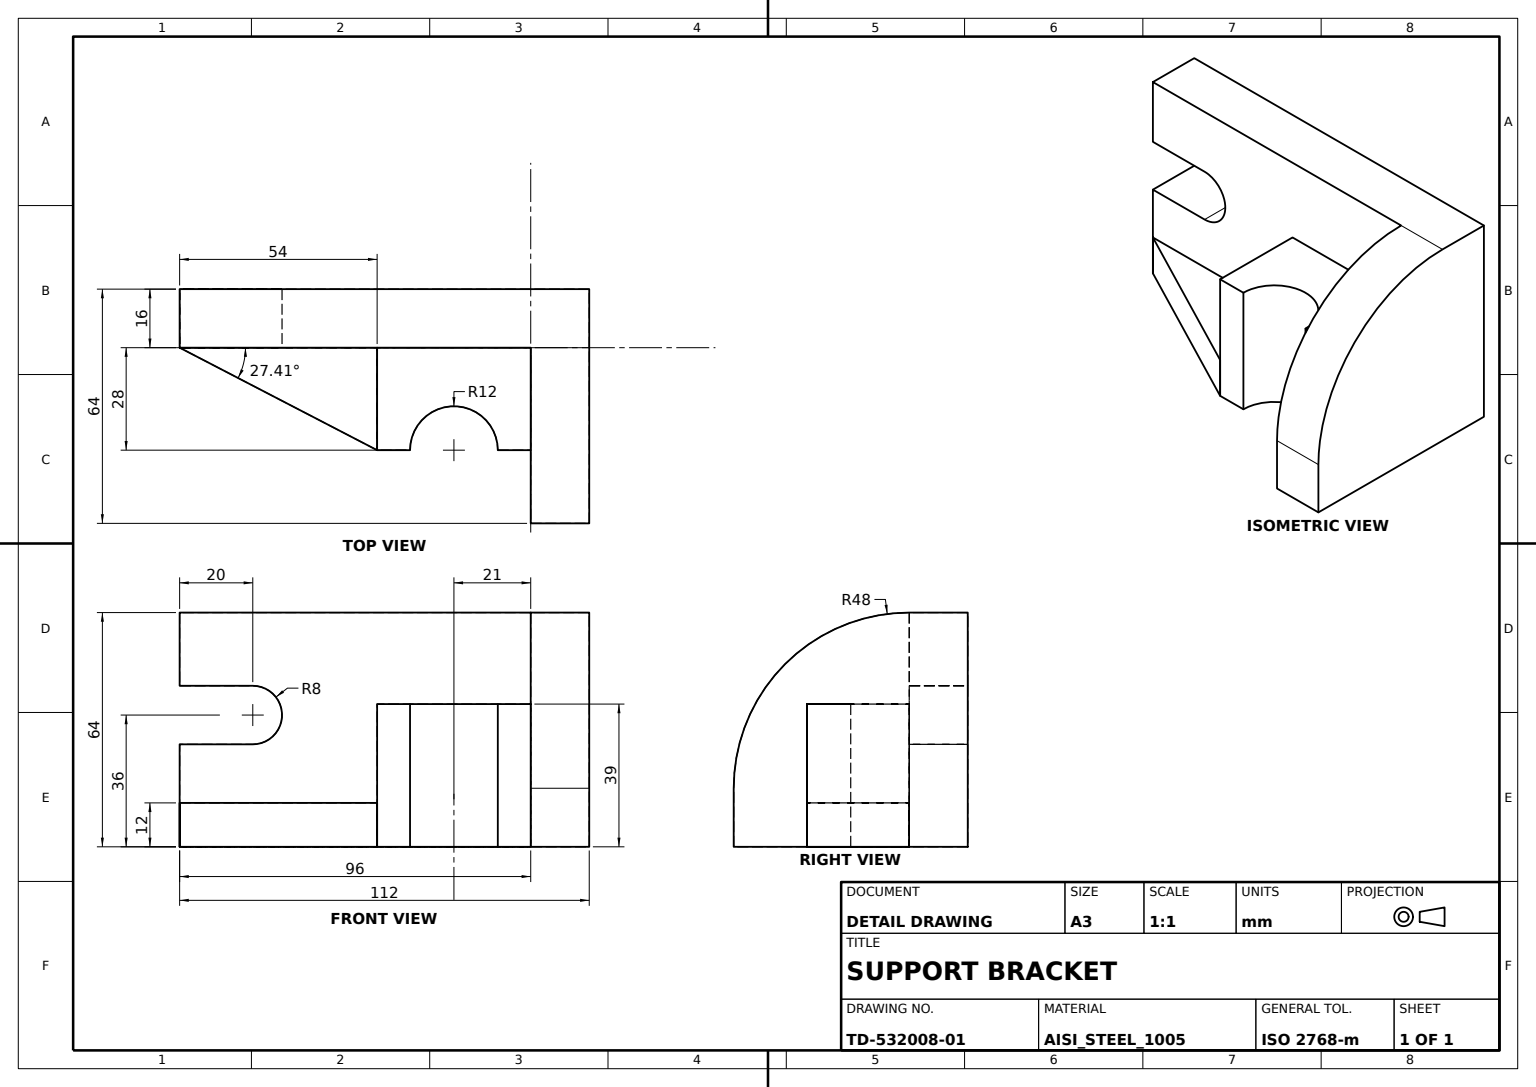
ISO-10303-21;
HEADER;
FILE_DESCRIPTION((''),'2;1');
FILE_NAME('','',(''),(''),'','','');
FILE_SCHEMA(('AUTOMOTIVE_DESIGN'));
ENDSEC;
DATA;
#1=APPLICATION_CONTEXT('');
#2=PRODUCT_CONTEXT('',#1,'mechanical');
#3=PRODUCT('','','',(#2));
#4=PRODUCT_DEFINITION_FORMATION('','',#3);
#5=PRODUCT_DEFINITION_CONTEXT('',#1,'design');
#6=PRODUCT_DEFINITION('','',#4,#5);
#7=PRODUCT_DEFINITION_SHAPE('','',#6);
#8=(LENGTH_UNIT()NAMED_UNIT(*)SI_UNIT(.MILLI.,.METRE.));
#9=(NAMED_UNIT(*)PLANE_ANGLE_UNIT()SI_UNIT($,.RADIAN.));
#10=(NAMED_UNIT(*)SI_UNIT($,.STERADIAN.)SOLID_ANGLE_UNIT());
#11=UNCERTAINTY_MEASURE_WITH_UNIT(LENGTH_MEASURE(0.005),#8,'distance_accuracy_value','');
#12=(GEOMETRIC_REPRESENTATION_CONTEXT(3)GLOBAL_UNCERTAINTY_ASSIGNED_CONTEXT((#11))GLOBAL_UNIT_ASSIGNED_CONTEXT((#8,#9,#10))REPRESENTATION_CONTEXT('',''));
#13=CARTESIAN_POINT('',(16.,0.,64.));
#14=VERTEX_POINT('',#13);
#15=CARTESIAN_POINT('',(0.,0.,64.));
#16=VERTEX_POINT('',#15);
#17=DIRECTION('',(-1.,0.,0.));
#18=VECTOR('',#17,1000.);
#19=LINE('',#13,#18);
#20=EDGE_CURVE('',#14,#16,#19,.T.);
#21=ORIENTED_EDGE('',*,*,#20,.T.);
#22=CARTESIAN_POINT('',(0.,0.,44.));
#23=VERTEX_POINT('',#22);
#24=CARTESIAN_POINT('',(0.,0.,0.));
#25=DIRECTION('',(0.,0.,1.));
#26=VECTOR('',#25,1000.);
#27=LINE('',#24,#26);
#28=EDGE_CURVE('',#23,#16,#27,.T.);
#29=ORIENTED_EDGE('',*,*,#28,.F.);
#30=CARTESIAN_POINT('',(16.,0.,44.));
#31=VERTEX_POINT('',#30);
#32=DIRECTION('',(1.,0.,0.));
#33=VECTOR('',#32,1000.);
#34=LINE('',#22,#33);
#35=EDGE_CURVE('',#23,#31,#34,.T.);
#36=ORIENTED_EDGE('',*,*,#35,.T.);
#37=CARTESIAN_POINT('',(16.,0.,0.));
#38=LINE('',#37,#26);
#39=EDGE_CURVE('',#31,#14,#38,.T.);
#40=ORIENTED_EDGE('',*,*,#39,.T.);
#41=EDGE_LOOP('',(#21,#29,#36,#40));
#42=FACE_BOUND('',#41,.T.);
#43=DIRECTION('',(0.,-1.,0.));
#44=DIRECTION('',(0.,0.,-1.));
#45=AXIS2_PLACEMENT_3D('',#37,#43,#44);
#46=PLANE('',#45);
#47=ADVANCED_FACE('',(#42),#46,.T.);
#48=CARTESIAN_POINT('',(64.,112.,0.));
#49=VERTEX_POINT('',#48);
#50=CARTESIAN_POINT('',(0.,112.,0.));
#51=VERTEX_POINT('',#50);
#52=LINE('',#48,#18);
#53=EDGE_CURVE('',#49,#51,#52,.T.);
#54=ORIENTED_EDGE('',*,*,#53,.F.);
#55=CARTESIAN_POINT('',(64.,96.,0.));
#56=VERTEX_POINT('',#55);
#57=VECTOR('',#43,1000.);
#58=LINE('',#48,#57);
#59=EDGE_CURVE('',#49,#56,#58,.T.);
#60=ORIENTED_EDGE('',*,*,#59,.T.);
#61=CARTESIAN_POINT('',(16.,96.,0.));
#62=VERTEX_POINT('',#61);
#63=LINE('',#55,#18);
#64=EDGE_CURVE('',#56,#62,#63,.T.);
#65=ORIENTED_EDGE('',*,*,#64,.T.);
#66=VERTEX_POINT('',#37);
#67=LINE('',#61,#57);
#68=EDGE_CURVE('',#62,#66,#67,.T.);
#69=ORIENTED_EDGE('',*,*,#68,.T.);
#70=VERTEX_POINT('',#24);
#71=LINE('',#37,#18);
#72=EDGE_CURVE('',#66,#70,#71,.T.);
#73=ORIENTED_EDGE('',*,*,#72,.T.);
#74=CARTESIAN_POINT('',(0.,96.,0.));
#75=LINE('',#74,#57);
#76=EDGE_CURVE('',#51,#70,#75,.T.);
#77=ORIENTED_EDGE('',*,*,#76,.F.);
#78=EDGE_LOOP('',(#54,#60,#65,#69,#73,#77));
#79=FACE_BOUND('',#78,.T.);
#80=AXIS2_PLACEMENT_3D('',#61,#44,#17);
#81=PLANE('',#80);
#82=ADVANCED_FACE('',(#79),#81,.T.);
#83=CARTESIAN_POINT('',(16.,20.,44.));
#84=VERTEX_POINT('',#83);
#85=LINE('',#83,#57);
#86=EDGE_CURVE('',#84,#31,#85,.T.);
#87=ORIENTED_EDGE('',*,*,#86,.T.);
#88=ORIENTED_EDGE('',*,*,#35,.F.);
#89=CARTESIAN_POINT('',(0.,20.,44.));
#90=VERTEX_POINT('',#89);
#91=LINE('',#89,#57);
#92=EDGE_CURVE('',#90,#23,#91,.T.);
#93=ORIENTED_EDGE('',*,*,#92,.F.);
#94=LINE('',#89,#33);
#95=EDGE_CURVE('',#84,#90,#94,.F.);
#96=ORIENTED_EDGE('',*,*,#95,.F.);
#97=EDGE_LOOP('',(#87,#88,#93,#96));
#98=FACE_BOUND('',#97,.T.);
#99=AXIS2_PLACEMENT_3D('',#89,#25,#32);
#100=PLANE('',#99);
#101=ADVANCED_FACE('',(#98),#100,.F.);
#102=CARTESIAN_POINT('',(16.,20.,28.));
#103=VERTEX_POINT('',#102);
#104=CARTESIAN_POINT('',(16.,20.,36.));
#105=AXIS2_PLACEMENT_3D('',#104,#32,#43);
#106=CIRCLE('',#105,8.);
#107=EDGE_CURVE('',#103,#84,#106,.T.);
#108=ORIENTED_EDGE('',*,*,#107,.F.);
#109=CARTESIAN_POINT('',(16.,0.,28.));
#110=VERTEX_POINT('',#109);
#111=DIRECTION('',(0.,1.,0.));
#112=VECTOR('',#111,1000.);
#113=LINE('',#109,#112);
#114=EDGE_CURVE('',#110,#103,#113,.T.);
#115=ORIENTED_EDGE('',*,*,#114,.F.);
#116=EDGE_CURVE('',#66,#110,#38,.T.);
#117=ORIENTED_EDGE('',*,*,#116,.F.);
#118=ORIENTED_EDGE('',*,*,#68,.F.);
#119=CARTESIAN_POINT('',(16.,96.,64.));
#120=VERTEX_POINT('',#119);
#121=VECTOR('',#44,1000.);
#122=LINE('',#119,#121);
#123=EDGE_CURVE('',#120,#62,#122,.T.);
#124=ORIENTED_EDGE('',*,*,#123,.F.);
#125=LINE('',#13,#112);
#126=EDGE_CURVE('',#14,#120,#125,.T.);
#127=ORIENTED_EDGE('',*,*,#126,.F.);
#128=ORIENTED_EDGE('',*,*,#39,.F.);
#129=ORIENTED_EDGE('',*,*,#86,.F.);
#130=EDGE_LOOP('',(#108,#115,#117,#118,#124,#127,#128,#129));
#131=FACE_BOUND('',#130,.T.);
#132=AXIS2_PLACEMENT_3D('',#37,#17,#25);
#133=PLANE('',#132);
#134=ADVANCED_FACE('',(#131),#133,.F.);
#135=CARTESIAN_POINT('',(0.,0.,28.));
#136=VERTEX_POINT('',#135);
#137=EDGE_CURVE('',#70,#136,#27,.T.);
#138=ORIENTED_EDGE('',*,*,#137,.F.);
#139=ORIENTED_EDGE('',*,*,#72,.F.);
#140=ORIENTED_EDGE('',*,*,#116,.T.);
#141=LINE('',#135,#33);
#142=EDGE_CURVE('',#136,#110,#141,.T.);
#143=ORIENTED_EDGE('',*,*,#142,.F.);
#144=EDGE_LOOP('',(#138,#139,#140,#143));
#145=FACE_BOUND('',#144,.T.);
#146=ADVANCED_FACE('',(#145),#46,.T.);
#147=ORIENTED_EDGE('',*,*,#123,.T.);
#148=ORIENTED_EDGE('',*,*,#64,.F.);
#149=CARTESIAN_POINT('',(64.,96.,16.));
#150=VERTEX_POINT('',#149);
#151=CARTESIAN_POINT('',(64.,96.,64.));
#152=LINE('',#151,#121);
#153=EDGE_CURVE('',#150,#56,#152,.T.);
#154=ORIENTED_EDGE('',*,*,#153,.F.);
#155=CARTESIAN_POINT('',(16.,96.,16.));
#156=AXIS2_PLACEMENT_3D('',#155,#111,#25);
#157=CIRCLE('',#156,48.);
#158=EDGE_CURVE('',#150,#120,#157,.F.);
#159=ORIENTED_EDGE('',*,*,#158,.T.);
#160=EDGE_LOOP('',(#147,#148,#154,#159));
#161=FACE_BOUND('',#160,.T.);
#162=AXIS2_PLACEMENT_3D('',#74,#111,#25);
#163=PLANE('',#162);
#164=ADVANCED_FACE('',(#161),#163,.F.);
#165=ORIENTED_EDGE('',*,*,#59,.F.);
#166=CARTESIAN_POINT('',(64.,112.,16.));
#167=VERTEX_POINT('',#166);
#168=CARTESIAN_POINT('',(64.,112.,64.));
#169=LINE('',#168,#121);
#170=EDGE_CURVE('',#167,#49,#169,.T.);
#171=ORIENTED_EDGE('',*,*,#170,.F.);
#172=LINE('',#149,#57);
#173=EDGE_CURVE('',#167,#150,#172,.T.);
#174=ORIENTED_EDGE('',*,*,#173,.T.);
#175=ORIENTED_EDGE('',*,*,#153,.T.);
#176=EDGE_LOOP('',(#165,#171,#174,#175));
#177=FACE_BOUND('',#176,.T.);
#178=AXIS2_PLACEMENT_3D('',#168,#17,#25);
#179=PLANE('',#178);
#180=ADVANCED_FACE('',(#177),#179,.F.);
#181=ORIENTED_EDGE('',*,*,#142,.T.);
#182=ORIENTED_EDGE('',*,*,#114,.T.);
#183=CARTESIAN_POINT('',(0.,20.,28.));
#184=VERTEX_POINT('',#183);
#185=LINE('',#183,#33);
#186=EDGE_CURVE('',#103,#184,#185,.F.);
#187=ORIENTED_EDGE('',*,*,#186,.T.);
#188=LINE('',#135,#112);
#189=EDGE_CURVE('',#136,#184,#188,.T.);
#190=ORIENTED_EDGE('',*,*,#189,.F.);
#191=EDGE_LOOP('',(#181,#182,#187,#190));
#192=FACE_BOUND('',#191,.T.);
#193=AXIS2_PLACEMENT_3D('',#135,#44,#111);
#194=PLANE('',#193);
#195=ADVANCED_FACE('',(#192),#194,.F.);
#196=CARTESIAN_POINT('',(16.,112.,64.));
#197=VERTEX_POINT('',#196);
#198=LINE('',#196,#57);
#199=EDGE_CURVE('',#120,#197,#198,.F.);
#200=ORIENTED_EDGE('',*,*,#199,.F.);
#201=ORIENTED_EDGE('',*,*,#158,.F.);
#202=ORIENTED_EDGE('',*,*,#173,.F.);
#203=CARTESIAN_POINT('',(16.,112.,16.));
#204=AXIS2_PLACEMENT_3D('',#203,#111,#25);
#205=CIRCLE('',#204,48.);
#206=EDGE_CURVE('',#197,#167,#205,.T.);
#207=ORIENTED_EDGE('',*,*,#206,.F.);
#208=EDGE_LOOP('',(#200,#201,#202,#207));
#209=FACE_BOUND('',#208,.T.);
#210=CYLINDRICAL_SURFACE('',#204,48.);
#211=ADVANCED_FACE('',(#209),#210,.T.);
#212=ORIENTED_EDGE('',*,*,#170,.T.);
#213=ORIENTED_EDGE('',*,*,#53,.T.);
#214=CARTESIAN_POINT('',(0.,112.,64.));
#215=VERTEX_POINT('',#214);
#216=LINE('',#50,#26);
#217=EDGE_CURVE('',#51,#215,#216,.T.);
#218=ORIENTED_EDGE('',*,*,#217,.T.);
#219=LINE('',#214,#33);
#220=EDGE_CURVE('',#215,#197,#219,.T.);
#221=ORIENTED_EDGE('',*,*,#220,.T.);
#222=ORIENTED_EDGE('',*,*,#206,.T.);
#223=EDGE_LOOP('',(#212,#213,#218,#221,#222));
#224=FACE_BOUND('',#223,.T.);
#225=AXIS2_PLACEMENT_3D('',#50,#111,#25);
#226=PLANE('',#225);
#227=ADVANCED_FACE('',(#224),#226,.T.);
#228=ORIENTED_EDGE('',*,*,#220,.F.);
#229=LINE('',#15,#112);
#230=EDGE_CURVE('',#16,#215,#229,.T.);
#231=ORIENTED_EDGE('',*,*,#230,.F.);
#232=ORIENTED_EDGE('',*,*,#20,.F.);
#233=ORIENTED_EDGE('',*,*,#126,.T.);
#234=ORIENTED_EDGE('',*,*,#199,.T.);
#235=EDGE_LOOP('',(#228,#231,#232,#233,#234));
#236=FACE_BOUND('',#235,.T.);
#237=AXIS2_PLACEMENT_3D('',#13,#25,#43);
#238=PLANE('',#237);
#239=ADVANCED_FACE('',(#236),#238,.T.);
#240=ORIENTED_EDGE('',*,*,#230,.T.);
#241=ORIENTED_EDGE('',*,*,#217,.F.);
#242=ORIENTED_EDGE('',*,*,#76,.T.);
#243=ORIENTED_EDGE('',*,*,#137,.T.);
#244=ORIENTED_EDGE('',*,*,#189,.T.);
#245=CARTESIAN_POINT('',(0.,20.,36.));
#246=AXIS2_PLACEMENT_3D('',#245,#32,#43);
#247=CIRCLE('',#246,8.);
#248=EDGE_CURVE('',#184,#90,#247,.T.);
#249=ORIENTED_EDGE('',*,*,#248,.T.);
#250=ORIENTED_EDGE('',*,*,#92,.T.);
#251=ORIENTED_EDGE('',*,*,#28,.T.);
#252=EDGE_LOOP('',(#240,#241,#242,#243,#244,#249,#250,#251));
#253=FACE_BOUND('',#252,.T.);
#254=AXIS2_PLACEMENT_3D('',#24,#17,#25);
#255=PLANE('',#254);
#256=ADVANCED_FACE('',(#253),#255,.T.);
#257=ORIENTED_EDGE('',*,*,#186,.F.);
#258=ORIENTED_EDGE('',*,*,#107,.T.);
#259=ORIENTED_EDGE('',*,*,#95,.T.);
#260=ORIENTED_EDGE('',*,*,#248,.F.);
#261=EDGE_LOOP('',(#257,#258,#259,#260));
#262=FACE_BOUND('',#261,.T.);
#263=AXIS2_PLACEMENT_3D('',#245,#32,#44);
#264=CYLINDRICAL_SURFACE('',#263,8.);
#265=ADVANCED_FACE('',(#262),#264,.F.);
#266=CLOSED_SHELL('',(#47,#82,#101,#134,#146,#164,#180,#195,#211,#227,#239,#256,#265));
#267=MANIFOLD_SOLID_BREP('',#266);
#268=CARTESIAN_POINT('',(16.,54.,0.));
#269=VERTEX_POINT('',#268);
#270=VERTEX_POINT('',#61);
#271=LINE('',#268,#112);
#272=EDGE_CURVE('',#269,#270,#271,.T.);
#273=ORIENTED_EDGE('',*,*,#272,.T.);
#274=CARTESIAN_POINT('',(44.,96.,0.));
#275=VERTEX_POINT('',#274);
#276=LINE('',#274,#18);
#277=EDGE_CURVE('',#275,#270,#276,.T.);
#278=ORIENTED_EDGE('',*,*,#277,.F.);
#279=CARTESIAN_POINT('',(44.,87.,0.));
#280=VERTEX_POINT('',#279);
#281=CARTESIAN_POINT('',(44.,54.,0.));
#282=LINE('',#281,#112);
#283=EDGE_CURVE('',#280,#275,#282,.T.);
#284=ORIENTED_EDGE('',*,*,#283,.F.);
#285=CARTESIAN_POINT('',(44.,63.,0.));
#286=VERTEX_POINT('',#285);
#287=CARTESIAN_POINT('',(44.,75.,0.));
#288=AXIS2_PLACEMENT_3D('',#287,#25,#32);
#289=CIRCLE('',#288,12.);
#290=EDGE_CURVE('',#286,#280,#289,.F.);
#291=ORIENTED_EDGE('',*,*,#290,.F.);
#292=VERTEX_POINT('',#281);
#293=EDGE_CURVE('',#292,#286,#282,.T.);
#294=ORIENTED_EDGE('',*,*,#293,.F.);
#295=LINE('',#281,#18);
#296=EDGE_CURVE('',#292,#269,#295,.T.);
#297=ORIENTED_EDGE('',*,*,#296,.T.);
#298=EDGE_LOOP('',(#273,#278,#284,#291,#294,#297));
#299=FACE_BOUND('',#298,.T.);
#300=AXIS2_PLACEMENT_3D('',#281,#25,#32);
#301=PLANE('',#300);
#302=ADVANCED_FACE('',(#299),#301,.F.);
#303=CARTESIAN_POINT('',(44.,63.,39.));
#304=VERTEX_POINT('',#303);
#305=CARTESIAN_POINT('',(44.,54.,39.));
#306=VERTEX_POINT('',#305);
#307=CARTESIAN_POINT('',(44.,96.,39.));
#308=LINE('',#307,#57);
#309=EDGE_CURVE('',#304,#306,#308,.T.);
#310=ORIENTED_EDGE('',*,*,#309,.T.);
#311=LINE('',#305,#121);
#312=EDGE_CURVE('',#306,#292,#311,.T.);
#313=ORIENTED_EDGE('',*,*,#312,.T.);
#314=ORIENTED_EDGE('',*,*,#293,.T.);
#315=CARTESIAN_POINT('',(44.,63.,-54961.));
#316=LINE('',#315,#26);
#317=EDGE_CURVE('',#304,#286,#316,.F.);
#318=ORIENTED_EDGE('',*,*,#317,.F.);
#319=EDGE_LOOP('',(#310,#313,#314,#318));
#320=FACE_BOUND('',#319,.T.);
#321=CARTESIAN_POINT('',(44.,0.,0.));
#322=AXIS2_PLACEMENT_3D('',#321,#32,#44);
#323=PLANE('',#322);
#324=ADVANCED_FACE('',(#320),#323,.T.);
#325=ORIENTED_EDGE('',*,*,#296,.F.);
#326=ORIENTED_EDGE('',*,*,#312,.F.);
#327=CARTESIAN_POINT('',(16.,54.,39.));
#328=VERTEX_POINT('',#327);
#329=LINE('',#305,#18);
#330=EDGE_CURVE('',#306,#328,#329,.T.);
#331=ORIENTED_EDGE('',*,*,#330,.T.);
#332=LINE('',#327,#121);
#333=EDGE_CURVE('',#328,#269,#332,.T.);
#334=ORIENTED_EDGE('',*,*,#333,.T.);
#335=EDGE_LOOP('',(#325,#326,#331,#334));
#336=FACE_BOUND('',#335,.T.);
#337=AXIS2_PLACEMENT_3D('',#305,#111,#25);
#338=PLANE('',#337);
#339=ADVANCED_FACE('',(#336),#338,.F.);
#340=CARTESIAN_POINT('',(16.,96.,39.));
#341=VERTEX_POINT('',#340);
#342=LINE('',#340,#57);
#343=EDGE_CURVE('',#341,#328,#342,.T.);
#344=ORIENTED_EDGE('',*,*,#343,.F.);
#345=LINE('',#61,#26);
#346=EDGE_CURVE('',#270,#341,#345,.T.);
#347=ORIENTED_EDGE('',*,*,#346,.F.);
#348=ORIENTED_EDGE('',*,*,#272,.F.);
#349=ORIENTED_EDGE('',*,*,#333,.F.);
#350=EDGE_LOOP('',(#344,#347,#348,#349));
#351=FACE_BOUND('',#350,.T.);
#352=AXIS2_PLACEMENT_3D('',#37,#32,#44);
#353=PLANE('',#352);
#354=ADVANCED_FACE('',(#351),#353,.F.);
#355=VERTEX_POINT('',#307);
#356=LINE('',#307,#18);
#357=EDGE_CURVE('',#355,#341,#356,.T.);
#358=ORIENTED_EDGE('',*,*,#357,.F.);
#359=LINE('',#274,#26);
#360=EDGE_CURVE('',#275,#355,#359,.T.);
#361=ORIENTED_EDGE('',*,*,#360,.F.);
#362=ORIENTED_EDGE('',*,*,#277,.T.);
#363=ORIENTED_EDGE('',*,*,#346,.T.);
#364=EDGE_LOOP('',(#358,#361,#362,#363));
#365=FACE_BOUND('',#364,.T.);
#366=AXIS2_PLACEMENT_3D('',#274,#43,#44);
#367=PLANE('',#366);
#368=ADVANCED_FACE('',(#365),#367,.F.);
#369=CARTESIAN_POINT('',(44.,87.,39.));
#370=VERTEX_POINT('',#369);
#371=CARTESIAN_POINT('',(44.,87.,-54961.));
#372=LINE('',#371,#26);
#373=EDGE_CURVE('',#280,#370,#372,.T.);
#374=ORIENTED_EDGE('',*,*,#373,.T.);
#375=CARTESIAN_POINT('',(44.,75.,39.));
#376=AXIS2_PLACEMENT_3D('',#375,#25,#43);
#377=CIRCLE('',#376,12.);
#378=EDGE_CURVE('',#370,#304,#377,.T.);
#379=ORIENTED_EDGE('',*,*,#378,.T.);
#380=ORIENTED_EDGE('',*,*,#317,.T.);
#381=ORIENTED_EDGE('',*,*,#290,.T.);
#382=EDGE_LOOP('',(#374,#379,#380,#381));
#383=FACE_BOUND('',#382,.T.);
#384=CARTESIAN_POINT('',(44.,75.,-54961.));
#385=AXIS2_PLACEMENT_3D('',#384,#25,#32);
#386=CYLINDRICAL_SURFACE('',#385,12.);
#387=ADVANCED_FACE('',(#383),#386,.F.);
#388=EDGE_CURVE('',#355,#370,#308,.T.);
#389=ORIENTED_EDGE('',*,*,#388,.T.);
#390=ORIENTED_EDGE('',*,*,#373,.F.);
#391=ORIENTED_EDGE('',*,*,#283,.T.);
#392=ORIENTED_EDGE('',*,*,#360,.T.);
#393=EDGE_LOOP('',(#389,#390,#391,#392));
#394=FACE_BOUND('',#393,.T.);
#395=ADVANCED_FACE('',(#394),#323,.T.);
#396=ORIENTED_EDGE('',*,*,#343,.T.);
#397=ORIENTED_EDGE('',*,*,#330,.F.);
#398=ORIENTED_EDGE('',*,*,#309,.F.);
#399=ORIENTED_EDGE('',*,*,#378,.F.);
#400=ORIENTED_EDGE('',*,*,#388,.F.);
#401=ORIENTED_EDGE('',*,*,#357,.T.);
#402=EDGE_LOOP('',(#396,#397,#398,#399,#400,#401));
#403=FACE_BOUND('',#402,.T.);
#404=AXIS2_PLACEMENT_3D('',#307,#44,#17);
#405=PLANE('',#404);
#406=ADVANCED_FACE('',(#403),#405,.F.);
#407=CLOSED_SHELL('',(#302,#324,#339,#354,#368,#387,#395,#406));
#408=MANIFOLD_SOLID_BREP('',#407);
#409=CARTESIAN_POINT('',(16.,0.,12.));
#410=VERTEX_POINT('',#409);
#411=VERTEX_POINT('',#37);
#412=LINE('',#409,#121);
#413=EDGE_CURVE('',#410,#411,#412,.T.);
#414=ORIENTED_EDGE('',*,*,#413,.F.);
#415=CARTESIAN_POINT('',(16.,54.,12.));
#416=VERTEX_POINT('',#415);
#417=LINE('',#409,#112);
#418=EDGE_CURVE('',#410,#416,#417,.T.);
#419=ORIENTED_EDGE('',*,*,#418,.T.);
#420=VERTEX_POINT('',#268);
#421=LINE('',#415,#121);
#422=EDGE_CURVE('',#416,#420,#421,.T.);
#423=ORIENTED_EDGE('',*,*,#422,.T.);
#424=LINE('',#37,#112);
#425=EDGE_CURVE('',#411,#420,#424,.T.);
#426=ORIENTED_EDGE('',*,*,#425,.F.);
#427=EDGE_LOOP('',(#414,#419,#423,#426));
#428=FACE_BOUND('',#427,.T.);
#429=AXIS2_PLACEMENT_3D('',#409,#17,#25);
#430=PLANE('',#429);
#431=ADVANCED_FACE('',(#428),#430,.T.);
#432=ORIENTED_EDGE('',*,*,#418,.F.);
#433=CARTESIAN_POINT('',(44.,54.,12.));
#434=VERTEX_POINT('',#433);
#435=DIRECTION('',(-0.460317164,-0.887754531,0.));
#436=VECTOR('',#435,1000.);
#437=LINE('',#433,#436);
#438=EDGE_CURVE('',#434,#410,#437,.T.);
#439=ORIENTED_EDGE('',*,*,#438,.F.);
#440=LINE('',#415,#33);
#441=EDGE_CURVE('',#416,#434,#440,.T.);
#442=ORIENTED_EDGE('',*,*,#441,.F.);
#443=EDGE_LOOP('',(#432,#439,#442));
#444=FACE_BOUND('',#443,.T.);
#445=CARTESIAN_POINT('',(0.,0.,12.));
#446=AXIS2_PLACEMENT_3D('',#445,#44,#17);
#447=PLANE('',#446);
#448=ADVANCED_FACE('',(#444),#447,.F.);
#449=VERTEX_POINT('',#281);
#450=LINE('',#281,#436);
#451=EDGE_CURVE('',#449,#411,#450,.T.);
#452=ORIENTED_EDGE('',*,*,#451,.F.);
#453=LINE('',#433,#121);
#454=EDGE_CURVE('',#434,#449,#453,.T.);
#455=ORIENTED_EDGE('',*,*,#454,.F.);
#456=ORIENTED_EDGE('',*,*,#438,.T.);
#457=ORIENTED_EDGE('',*,*,#413,.T.);
#458=EDGE_LOOP('',(#452,#455,#456,#457));
#459=FACE_BOUND('',#458,.T.);
#460=DIRECTION('',(0.887754531,-0.460317164,0.));
#461=DIRECTION('',(0.460317164,0.887754531,0.));
#462=AXIS2_PLACEMENT_3D('',#433,#460,#461);
#463=PLANE('',#462);
#464=ADVANCED_FACE('',(#459),#463,.T.);
#465=ORIENTED_EDGE('',*,*,#422,.F.);
#466=ORIENTED_EDGE('',*,*,#441,.T.);
#467=ORIENTED_EDGE('',*,*,#454,.T.);
#468=LINE('',#268,#33);
#469=EDGE_CURVE('',#420,#449,#468,.T.);
#470=ORIENTED_EDGE('',*,*,#469,.F.);
#471=EDGE_LOOP('',(#465,#466,#467,#470));
#472=FACE_BOUND('',#471,.T.);
#473=AXIS2_PLACEMENT_3D('',#415,#111,#17);
#474=PLANE('',#473);
#475=ADVANCED_FACE('',(#472),#474,.T.);
#476=ORIENTED_EDGE('',*,*,#425,.T.);
#477=ORIENTED_EDGE('',*,*,#469,.T.);
#478=ORIENTED_EDGE('',*,*,#451,.T.);
#479=EDGE_LOOP('',(#476,#477,#478));
#480=FACE_BOUND('',#479,.T.);
#481=AXIS2_PLACEMENT_3D('',#24,#44,#17);
#482=PLANE('',#481);
#483=ADVANCED_FACE('',(#480),#482,.T.);
#484=CLOSED_SHELL('',(#431,#448,#464,#475,#483));
#485=MANIFOLD_SOLID_BREP('',#484);
#486=ADVANCED_BREP_SHAPE_REPRESENTATION('',(#267,#408,#485),#12);
#487=SHAPE_DEFINITION_REPRESENTATION(#7,#486);
ENDSEC;
END-ISO-10303-21;
